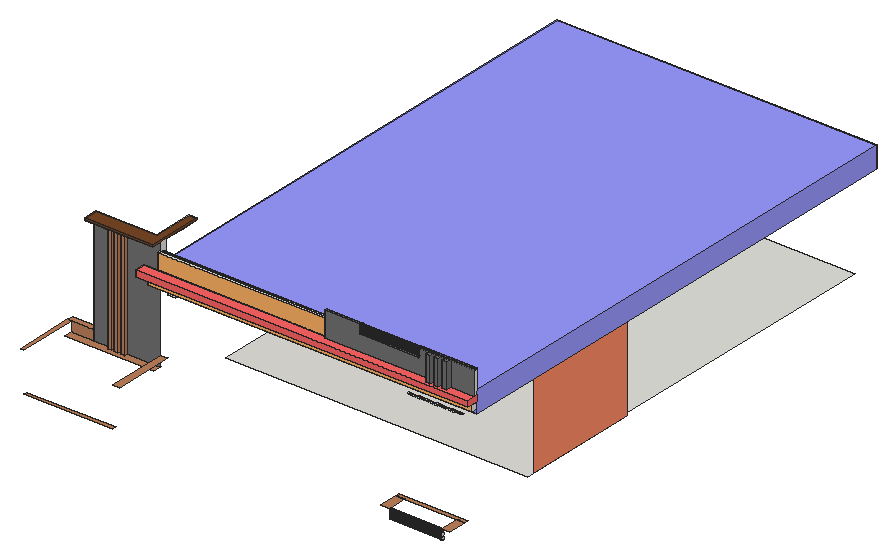
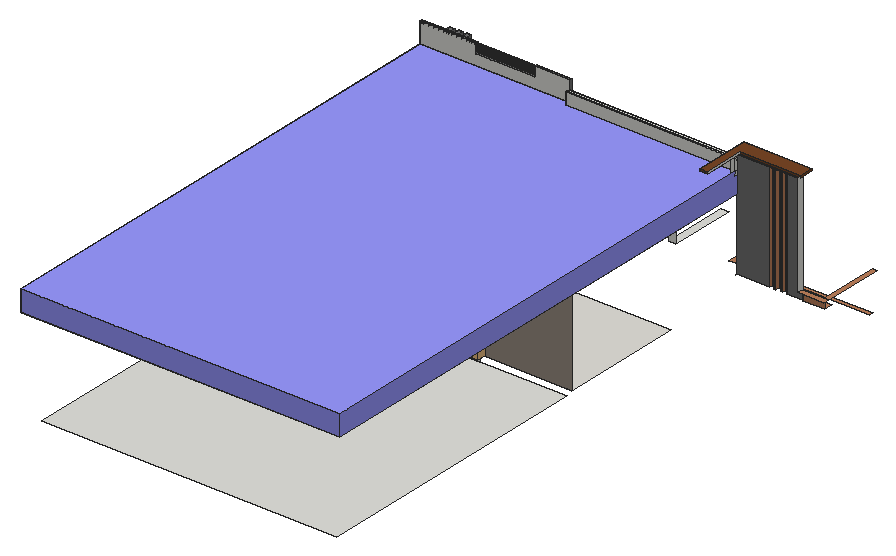
# SketchUp Ruby script. Lengths in inches.
U = 1.inch
M = Sketchup.active_model
def pt(a) = Geom::Point3d.new(a.map { |v| v * U })
def face(e, loops, mat)
  f = e.add_face(loops[0].map { |a| pt(a) })
  loops[1..].each { |l| e.add_face(l.map { |a| pt(a) }).erase! }
  f.material = f.back_material = mat if mat
  f
end
# faces: each face lists its corners as indices into pts; further lists are holes
def faces(e, pts, list, mat = nil) = list.each { |f| face(e, (f[0].is_a?(Array) ? f : [f]).map { |l| l.map { |i| pts[i] } }, mat) }
# xy, xz, yz: faces in a plane at the given z, y or x. An outline is a flat list of corners, or four numbers for a rectangle; further outlines are holes
def ring(l) = l.size == 4 ? [[l[0], l[1]], [l[2], l[1]], [l[2], l[3]], [l[0], l[3]]] : l.each_slice(2).to_a
def flat(e, list, mat, &to3) = list.each { |f| face(e, (f[0].is_a?(Array) ? f : [f]).map { |l| ring(l).map { |u, v| to3.(u, v) } }, mat) }
def xy(e, z, list, mat = nil) = flat(e, list, mat) { |x, y| [x, y, z] }
def xz(e, y, list, mat = nil) = flat(e, list, mat) { |x, z| [x, y, z] }
def yz(e, x, list, mat = nil) = flat(e, list, mat) { |y, z| [x, y, z] }
def lines(e, pts, list) = list.each { |a, b| e.add_line(pt(pts[a]), pt(pts[b])) }
# prism: a flat outline (further loops are holes) pulled along v
def prism(e, loops, v, mat = nil)
  f = face(e, loops, mat); d = Geom::Vector3d.new(v.map { |x| x * U })
  f.pushpull(f.normal.samedirection?(d) ? d.length : -d.length)
end
def box(e, o, s, mat = nil) = prism(e, [[o, [o[0] + s[0], o[1], o[2]], [o[0] + s[0], o[1] + s[1], o[2]], [o[0], o[1] + s[1], o[2]]]], [0, 0, s[2]], mat)
def at(x, y, z, deg = 0) = Geom::Transformation.translation(pt([x, y, z])) * Geom::Transformation.rotation(ORIGIN, Z_AXIS, deg.degrees)
def axes(o, x, y, z) = Geom::Transformation.new([*x, 0, *y, 0, *z, 0, *pt(o).to_a, 1])
def part(name) = M.definitions.add(name)
# library, detail: a bought-in or finely detailed component or shape, given as its bounding box
def library(name, o, s) = part(name).tap { |d| box(d.entities, o, s) }
def detail(e, o, s) = box(e.add_group.entities, o, s)
def put(e, d, t, mat = nil) = e.add_instance(d, t).tap { |i| i.material = mat if mat }
def group(e, t, mat = nil) = e.add_group.tap { |g| g.transformation = t; g.material = mat if mat }.entities
root = M.entities
M.materials.add("[Color A03]").color = [255, 101, 101]
M.materials.add("[Color B03]").color = [255, 140, 101]
M.materials.add("[Color C03]").color = [255, 178, 101]
M.materials.add("[Color I02]").color = [153, 153, 255]
M.materials.add("[Color M05]").color = [114, 114, 114]
M.materials.add("[Marble Carrara Gold Floor Tile]").color = [225, 223, 217]
M.materials.add("[Translucent Glass Gray]1").color = [128, 128, 128]
M.materials["[Translucent Glass Gray]1"].alpha = 0.5
M.materials.add("[Water Stream Shallow]").color = [155, 145, 133]
M.materials.add("[Wood Cherry Original]").color = [152, 86, 42]
M.materials.add("[Wood Veneer 01]").color = [120, 70, 37]
M.materials.add("[Wood Veneer 02]").color = [190, 128, 91]
c1 = library("DOOR (1)",[0,-8.625,0],[36,11.25,84])
c2 = part("Group\#4")
xy(c2.entities,0,[[0,0,32.48,1.97]])
xy(c2.entities,0.98,[[0.98,0,31.5,0.98],[0.98,0.98,31.5,1.97]])
xy(c2.entities,8.86,[[0.98,0,31.5,0.98],[0.98,0.98,31.5,1.97]])
xy(c2.entities,9.84,[[0,0,32.48,1.97]])
xz(c2.entities,0,[[[0,0,32.48,9.84],[0.98,0.98,31.5,8.86]]])
xz(c2.entities,0.98,[[0.98,0.98,31.5,8.86]],"[Translucent Glass Gray]1")
xz(c2.entities,1.97,[[[0,0,32.48,9.84],[0.98,0.98,31.5,8.86]]])
yz(c2.entities,0,[[0,0,1.97,9.84]])
yz(c2.entities,0.98,[[0,0.98,0.98,8.86],[0.98,0.98,1.97,8.86]])
yz(c2.entities,31.5,[[0,0.98,0.98,8.86],[0.98,0.98,1.97,8.86]])
yz(c2.entities,32.48,[[0,0,1.97,9.84]])
c3 = part("Group\#6")
xy(c3.entities,0,[[0,0,32.48,1.97]])
xy(c3.entities,0.98,[[0.98,0,31.5,0.98],[0.98,0.98,31.5,1.97]])
xy(c3.entities,71.85,[[0.98,0,31.5,0.98],[0.98,0.98,31.5,1.97]])
xy(c3.entities,72.83,[[0,0,32.48,1.97]])
xz(c3.entities,0,[[[0,0,32.48,72.83],[0.98,0.98,31.5,71.85]]])
xz(c3.entities,0.98,[[0.98,0.98,31.5,71.85]],"[Translucent Glass Gray]1")
xz(c3.entities,1.97,[[[0,0,32.48,72.83],[0.98,0.98,31.5,71.85]]])
yz(c3.entities,0,[[0,0,1.97,72.83]])
yz(c3.entities,0.98,[[0,0.98,0.98,71.85],[0.98,0.98,1.97,71.85]])
yz(c3.entities,31.5,[[0,0.98,0.98,71.85],[0.98,0.98,1.97,71.85]])
yz(c3.entities,32.48,[[0,0,1.97,72.83]])
c4 = part("FIXED+GLASS+WINDOW+WITH+TRANSOM")
g1 = group(c4.entities,at(0,7.5625,-3.14))
xy(g1,0,[[0,-3.73,93.63,0]])
xy(g1,2.39,[[2.6,-3.73,45.52,-2.8],[48.12,-3.73,91.03,0],[2.6,-0.93,45.52,0]])
xy(g1,105.27,[[2.6,-3.73,45.52,0],[45.52,-3.73,48.12,0],[48.12,-3.73,91.03,0]])
xy(g1,107.66,[[0,-3.73,93.63,0]])
xz(g1,-3.73,[[[0,0,93.63,107.66],[2.6,2.39,45.52,105.27],[48.12,2.39,91.03,105.27]]])
xz(g1,0,[[[0,0,93.63,107.66],[2.6,2.39,45.52,105.27],[48.12,2.39,91.03,105.27]]])
yz(g1,0,[[-3.73,0,0,107.66]])
yz(g1,2.6,[[-3.73,2.39,0,90.92],[-3.73,93.31,0,105.27]])
yz(g1,45.52,[[-3.73,2.39,0,105.27]])
yz(g1,48.12,[[-3.73,2.39,0,105.27]])
yz(g1,91.03,[[-3.73,2.39,0,105.27]])
yz(g1,93.63,[[-3.73,0,0,107.66]])
g2 = group(g1,at(2.6,0,90.92))
box(g2,[0,-3.73,0],[88.43,3.73,2.39])
put(g1,c2,axes([2.6,-0.93,93.31],[1.32132,0,0],[0,-0.94801,0],[0,0,1.2154]))
put(g1,c2,axes([48.12,-0.93,93.31],[1.32132,0,0],[0,-0.94801,0],[0,0,1.2154]))
put(g1,c3,axes([2.6,-0.93,2.39],[1.32132,0,0],[0,-0.94801,0],[0,0,1.2154]))
put(g1,c3,axes([48.12,-0.93,2.39],[1.32132,0,0],[0,-0.94801,0],[0,0,1.2154]))
xy(root,5.125,[[4.34,0,104.79,4.19]],"[Wood Veneer 02]")
xy(root,11.625,[[114.76,294.58,448.89,619.58]])
xy(root,14.625,[[386.33,27.35,395.89,48.85]],"[Wood Veneer 02]")
xy(root,14.6875,[[386.33,48.85,464.58,53.1]],"[Wood Veneer 02]")
xy(root,14.91,[[455.01,27.35,464.58,48.85]],"[Wood Veneer 02]")
xy(root,15,[[113.7,148.58,455.7,148.58,455.7,288.58,248.89,288.58,248.89,294.58,212.89,294.58,212.89,288.58,113.7,288.58]],"[Marble Carrara Gold Floor Tile]")
xy(root,38.8125,[[4.34,57.44,104.79,57.44,104.79,67.36,104.7,67.36,104.7,66.64,67.79,66.64,67.79,63.64,63.1,63.64,63.1,66.64,59.98,66.64,59.98,63.64,55.29,63.64,55.29,66.64,52.61,66.64,52.61,63.64,47.91,63.64,47.91,66.64,29.5,66.64,29.5,67.36,4.34,67.36]],"[Wood Veneer 02]")
xy(root,41.07,[[327.66,288.58,375.66,294.58]])
xy(root,50,[[0,0,4.34,67.36],[104.79,0,112.66,67.32],[0,67.36,29.5,73.72]],"[Wood Veneer 02]")
xy(root,84,[[212.89,288.58,248.89,294.58]])
xy(root,89.07,[[327.66,288.58,375.66,294.58]])
xy(root,107.35,[[104.79,78.01,113.42,152.44]])
xy(root,120,[[[455.7,65.3,464.7,65.3,464.7,628.58,104.7,628.58,104.7,148.58,110.64,148.58,110.64,78.01,113.7,78.01,113.7,288.58,455.7,288.58],[113.7,294.58,455.7,619.58]],[104.7,66.64,106.01,73.72],[104.7,73.72,106.01,148.58],[106.01,73.72,110.64,148.58]])
xy(root,121.125,[[104.79,67.32,113.42,152.44]])
xy(root,124.36,[[99.19,57.01,466.06,63.01]])
xy(root,130.99,[[99.19,57.01,466.06,63.01]])
xy(root,132,[[89.58,51.01,466.14,63.01]],"[Wood Cherry Original]")
xy(root,138.625,[[415.41,54.01,420.69,60.01],[424.66,54.01,429.94,60.01],[433.91,54.01,439.19,60.01],[297.02,60.01,342.89,63.01],[342.89,60.01,466.08,63.01],
  [104.95,63.01,297.02,66.01],[104.95,66.01,297.02,68.39]])
xy(root,138.625,[[89.58,51.01,466.14,51.01,466.14,63.01,466.08,63.01,466.08,60.01,439.19,60.01,439.19,54.01,433.91,54.01,433.91,60.01,429.94,60.01,429.94,54.01,424.66,54.01,424.66,60.01,420.69,60.01,420.69,54.01,415.41,54.01,415.41,60.01,297.02,60.01,297.02,63.01,89.58,63.01]],"[Color A03]")
xy(root,156,[[335.91,60.01,403.1,63.01]],"[Color M05]")
xy(root,156.51,[[104.95,63.01,297.02,66.01],[104.95,66.01,297.02,68.39]])
xy(root,165.75,[[28.39,55.2,29.5,71.95],[29.5,55.2,47.91,66.64],[47.91,55.2,52.61,63.64],[52.61,55.2,55.29,66.64],[55.29,55.2,59.98,63.64],
  [59.98,55.2,63.1,66.64],[63.1,55.2,67.79,63.64],[67.79,55.2,106.01,66.64],[47.91,63.64,52.61,66.64],[55.29,63.64,59.98,66.64],
  [63.1,63.64,67.79,66.64],[29.5,66.64,106.01,71.95],[29.5,71.95,96.84,73.72],[96.84,71.95,106.01,73.72],[96.84,73.72,106.01,76.7],
  [96.84,76.7,106.01,102.95],[96.84,102.95,106.01,117.33]])
xy(root,166.75,[[415.41,54.01,420.69,60.01],[424.66,54.01,429.94,60.01],[433.91,54.01,439.19,60.01],[297.02,60.01,335.91,63.01],[403.1,60.01,466.08,63.01]],"[Color M05]")
xy(root,167.75,[[28.39,55.2,106.01,55.2,106.01,117.33,96.84,117.33,96.84,71.95,28.39,71.95]],"[Wood Veneer 01]")
xz(root,48.85,[[386.33,14.625,395.89,14.6875],[455.01,14.6875,464.58,14.91]])
xz(root,51.01,[[89.58,132,466.14,138.625]],"[Color A03]")
xz(root,54.01,[[415.41,138.625,420.69,166.75],[424.66,138.625,429.94,166.75],[433.91,138.625,439.19,166.75]],"[Color M05]")
xz(root,55.2,[[28.39,165.75,106.01,167.75]],"[Wood Veneer 01]")
xz(root,57.01,[[99.19,124.36,466.06,130.99]],"[Color C03]")
xz(root,60.01,[[415.41,138.625,420.69,166.75],[424.66,138.625,429.94,166.75],[433.91,138.625,439.19,166.75]])
xz(root,60.01,[[297.02,138.625,415.41,138.625,415.41,166.75,403.1,166.75,403.1,156,335.91,156,335.91,166.75,297.02,166.75],[420.69,138.625,424.66,166.75],[429.94,138.625,433.91,166.75],[439.19,138.625,466.08,166.75]],"[Color M05]")
xz(root,63.01,[[99.19,124.36,466.06,130.99],[89.58,132,104.95,138.625],[104.95,132,342.89,138.625],[342.89,132,466.14,138.625],[297.02,138.625,297.02,166.75,335.91,166.75,335.91,156,403.1,156,403.1,166.75,466.08,166.75,466.08,138.625]])
xz(root,63.01,[[104.95,138.625,297.02,156.51]],"[Color C03]")
xz(root,63.64,[[47.91,38.8125,52.61,165.75],[55.29,38.8125,59.98,165.75],[63.1,38.8125,67.79,165.75]],"[Wood Veneer 02]")
xz(root,66.64,[[29.5,38.8125,47.91,165.75],[52.61,38.8125,55.29,165.75],[59.98,38.8125,63.1,165.75],[67.79,38.8125,104.7,38.8125,104.7,120,106.01,120,106.01,165.75,67.79,165.75]],"[Color M05]")
xz(root,67.36,[[4.34,38.8125,29.5,50]],"[Wood Veneer 02]")
xz(root,68.39,[[104.95,138.625,297.02,156.51]])
xz(root,71.95,[[28.39,165.75,96.84,167.75]],"[Wood Veneer 01]")
xz(root,117.33,[[96.84,165.75,106.01,167.75]],"[Wood Veneer 01]")
xz(root,152.44,[[104.79,107.35,113.42,121.125]])
xz(root,288.58,[[[113.7,15,212.89,15,212.89,84,248.89,84,248.89,15,455.7,15,455.7,120,113.7,120],[327.66,41.07,375.66,89.07]]],"[Water Stream Shallow]")
xz(root,294.58,[[212.89,11.625,248.89,15]])
yz(root,28.39,[[55.2,165.75,71.95,167.75]],"[Wood Veneer 01]")
yz(root,29.5,[[66.64,38.8125,66.64,165.75,73.72,165.75,73.72,50,67.36,50,67.36,38.8125]])
yz(root,47.91,[[63.64,38.8125,66.64,165.75]],"[Wood Veneer 02]")
yz(root,52.61,[[63.64,38.8125,66.64,165.75]],"[Wood Veneer 02]")
yz(root,55.29,[[63.64,38.8125,66.64,165.75]],"[Wood Veneer 02]")
yz(root,59.98,[[63.64,38.8125,66.64,165.75]],"[Wood Veneer 02]")
yz(root,63.1,[[63.64,38.8125,66.64,165.75]],"[Wood Veneer 02]")
yz(root,67.79,[[63.64,38.8125,66.64,165.75]],"[Wood Veneer 02]")
yz(root,89.58,[[51.01,132,63.01,138.625]],"[Color A03]")
yz(root,96.84,[[71.95,165.75,117.33,167.75]])
yz(root,99.19,[[57.01,124.36,63.01,130.99]])
yz(root,104.95,[[63.01,138.625,68.39,144],[63.01,144,66.01,156.51],[66.01,144,68.39,156.51]])
yz(root,106.01,[[66.64,120,73.72,165.75]])
yz(root,106.01,[[55.2,165.75,117.33,167.75]],"[Wood Veneer 01]")
yz(root,212.89,[[288.58,15,294.58,84]])
yz(root,248.89,[[288.58,15,294.58,84]])
yz(root,297.02,[[63.01,138.625,66.01,144],[66.01,138.625,68.39,144],[63.01,144,66.01,156.51],[66.01,144,68.39,156.51]])
yz(root,297.02,[[60.01,138.625,63.01,166.75]],"[Color M05]")
yz(root,327.66,[[288.58,41.07,294.58,89.07]])
yz(root,335.91,[[[60.01,156,63.01,166.75],[61.38,164.68,61.125,164.71,60.88,164.8125,60.68,164.97,60.52,165.18,60.42,165.42,60.38,165.68,60.42,165.9375,60.52,166.18,60.68,166.39,60.88,166.55,61.125,166.65,61.38,166.68,61.64,166.65,61.88,166.55,62.09,166.39,62.25,166.18,62.35,165.9375,62.38,165.68,62.35,165.42,62.25,165.18,62.09,164.97,61.88,164.8125,61.64,164.71],[61.38,161.43,61.125,161.46,60.88,161.5625,60.68,161.72,60.52,161.93,60.42,162.17,60.38,162.43,60.42,162.6875,60.52,162.93,60.68,163.14,60.88,163.3,61.125,163.4,61.38,163.43,61.64,163.4,61.88,163.3,62.09,163.14,62.25,162.93,62.35,162.6875,62.38,162.43,62.35,162.17,62.25,161.93,62.09,161.72,61.88,161.5625,61.64,161.46],[61.38,157.68,61.125,157.71,60.88,157.8125,60.68,157.97,60.52,158.18,60.42,158.42,60.38,158.68,60.42,158.9375,60.52,159.18,60.68,159.39,60.88,159.55,61.125,159.65,61.38,159.68,61.64,159.65,61.88,159.55,62.09,159.39,62.25,159.18,62.35,158.9375,62.38,158.68,62.35,158.42,62.25,158.18,62.09,157.97,61.88,157.8125,61.64,157.71]]],"[Color M05]")
yz(root,375.66,[[288.58,41.07,294.58,89.07]])
yz(root,395.89,[[28.97,3.38,28.61,3.43,28.28,3.57,28,3.78,27.78,4.07,27.64,4.4,27.59,4.76,27.64,5.11,27.78,5.44,28,5.73,28.28,5.95,28.61,6.09,28.97,6.13,29.32,6.09,29.66,5.95,29.94,5.73,30.16,5.44,30.3,5.11,30.34,4.76,30.3,4.4,30.16,4.07,29.94,3.78,29.66,3.57,29.32,3.43],[28.97,7.19,28.61,7.24,28.28,7.38,28,7.6,27.78,7.88,27.64,8.21,27.59,8.57,27.64,8.93,27.78,9.26,28,9.54,28.28,9.76,28.61,9.9,28.97,9.94,29.32,9.9,29.66,9.76,29.94,9.54,30.16,9.26,30.3,8.93,30.34,8.57,30.3,8.21,30.16,7.88,29.94,7.6,29.66,7.38,29.32,7.24],[28.97,11.57,28.61,11.62,28.28,11.75,28,11.97,27.78,12.26,27.64,12.59,27.59,12.94,27.64,13.3,27.78,13.63,28,13.92,28.28,14.14,28.61,14.27,28.97,14.32,29.32,14.27,29.66,14.14,29.94,13.92,30.16,13.63,30.3,13.3,30.34,12.94,30.3,12.59,30.16,12.26,29.94,11.97,29.66,11.75,29.32,11.62]])
yz(root,403.1,[[[60.01,156,63.01,166.75],[61.38,161.43,61.64,161.46,61.88,161.5625,62.09,161.72,62.25,161.93,62.35,162.17,62.38,162.43,62.35,162.6875,62.25,162.93,62.09,163.14,61.88,163.3,61.64,163.4,61.38,163.43,61.125,163.4,60.88,163.3,60.68,163.14,60.52,162.93,60.42,162.6875,60.38,162.43,60.42,162.17,60.52,161.93,60.68,161.72,60.88,161.5625,61.125,161.46]]],"[Color M05]")
yz(root,404.16,[[61.38,157.68,61.64,157.71,61.88,157.8125,62.09,157.97,62.25,158.18,62.35,158.42,62.38,158.68,62.35,158.9375,62.25,159.18,62.09,159.39,61.88,159.55,61.64,159.65,61.38,159.68,61.125,159.65,60.88,159.55,60.68,159.39,60.52,159.18,60.42,158.9375,60.38,158.68,60.42,158.42,60.52,158.18,60.68,157.97,60.88,157.8125,61.125,157.71]])
yz(root,415.41,[[54.01,138.625,60.01,166.75]],"[Color M05]")
yz(root,420.69,[[54.01,138.625,60.01,166.75]],"[Color M05]")
yz(root,424.66,[[54.01,138.625,60.01,166.75]],"[Color M05]")
yz(root,429.94,[[54.01,138.625,60.01,166.75]],"[Color M05]")
yz(root,433.91,[[54.01,138.625,60.01,166.75]],"[Color M05]")
yz(root,439.19,[[54.01,138.625,60.01,166.75]],"[Color M05]")
yz(root,455.26,[[28.97,7.19,29.32,7.24,29.66,7.38,29.94,7.6,30.16,7.88,30.3,8.21,30.34,8.57,30.3,8.93,30.16,9.26,29.94,9.54,29.66,9.76,29.32,9.9,28.97,9.94,28.61,9.9,28.28,9.76,28,9.54,27.78,9.26,27.64,8.93,27.59,8.57,27.64,8.21,27.78,7.88,28,7.6,28.28,7.38,28.61,7.24]])
yz(root,455.51,[[28.97,3.38,29.32,3.43,29.66,3.57,29.94,3.78,30.16,4.07,30.3,4.4,30.34,4.76,30.3,5.11,30.16,5.44,29.94,5.73,29.66,5.95,29.32,6.09,28.97,6.13,28.61,6.09,28.28,5.95,28,5.73,27.78,5.44,27.64,5.11,27.59,4.76,27.64,4.4,27.78,4.07,28,3.78,28.28,3.57,28.61,3.43]])
yz(root,455.7,[[157.58,15,288.58,120]],"[Color B03]")
yz(root,466.06,[[57.01,124.36,63.01,130.99]])
yz(root,466.08,[[60.01,138.625,63.01,166.75]])
yz(root,466.14,[[61.38,164.68,61.64,164.71,61.88,164.8125,62.09,164.97,62.25,165.18,62.35,165.42,62.38,165.68,62.35,165.9375,62.25,166.18,62.09,166.39,61.88,166.55,61.64,166.65,61.38,166.68,61.125,166.65,60.88,166.55,60.68,166.39,60.52,166.18,60.42,165.9375,60.38,165.68,60.42,165.42,60.52,165.18,60.68,164.97,60.88,164.8125,61.125,164.71]])
yz(root,466.14,[[51.01,132,63.01,138.625]],"[Color A03]")
p = [[395.89,28.28,3.57],[395.89,28.61,3.43],[455.51,28.61,3.43],[455.51,28.28,3.57],[395.89,28.97,3.38],[455.51,28.97,3.38],
  [395.89,29.32,3.43],[455.51,29.32,3.43],[395.89,29.66,3.57],[455.51,29.66,3.57],[395.89,28,3.78],[455.51,28,3.78],
  [395.89,29.94,3.78],[455.51,29.94,3.78],[395.89,27.78,4.07],[455.51,27.78,4.07],[395.89,30.16,4.07],[455.51,30.16,4.07],
  [395.89,27.64,4.4],[455.51,27.64,4.4],[395.89,30.3,4.4],[455.51,30.3,4.4],[395.89,27.59,4.76],[455.51,27.59,4.76],
  [395.89,30.34,4.76],[455.51,30.34,4.76],[395.89,27.64,5.11],[455.51,27.64,5.11],[395.89,30.3,5.11],[455.51,30.3,5.11],
  [395.89,27.78,5.44],[455.51,27.78,5.44],[395.89,30.16,5.44],[455.51,30.16,5.44],[395.89,28,5.73],[455.51,28,5.73],
  [395.89,29.94,5.73],[455.51,29.94,5.73],[395.89,28.28,5.95],[455.51,28.28,5.95],[395.89,29.66,5.95],[455.51,29.66,5.95],
  [395.89,28.61,6.09],[455.51,28.61,6.09],[395.89,29.32,6.09],[455.51,29.32,6.09],[395.89,28.97,6.13],[455.51,28.97,6.13],
  [395.89,28.28,7.38],[395.89,28.61,7.24],[455.26,28.61,7.24],[455.26,28.28,7.38],[395.89,28.97,7.19],[455.26,28.97,7.19],
  [395.89,29.32,7.24],[455.26,29.32,7.24],[395.89,29.66,7.38],[455.26,29.66,7.38],[395.89,28,7.6],[455.26,28,7.6],
  [395.89,29.94,7.6],[455.26,29.94,7.6],[395.89,27.78,7.88],[455.26,27.78,7.88],[395.89,30.16,7.88],[455.26,30.16,7.88],
  [395.89,27.64,8.21],[455.26,27.64,8.21],[395.89,30.3,8.21],[455.26,30.3,8.21],[395.89,27.59,8.57],[455.26,27.59,8.57],
  [395.89,30.34,8.57],[455.26,30.34,8.57],[395.89,27.64,8.93],[455.26,27.64,8.93],[395.89,30.3,8.93],[455.26,30.3,8.93],
  [395.89,27.78,9.26],[455.26,27.78,9.26],[395.89,30.16,9.26],[455.26,30.16,9.26],[395.89,28,9.54],[455.26,28,9.54],
  [395.89,29.94,9.54],[455.26,29.94,9.54],[395.89,28.28,9.76],[455.26,28.28,9.76],[395.89,29.66,9.76],[455.26,29.66,9.76],
  [395.89,28.61,9.9],[455.26,28.61,9.9],[395.89,29.32,9.9],[455.26,29.32,9.9],[395.89,28.97,9.94],[455.26,28.97,9.94],
  [395.89,28.28,11.75],[395.89,28.61,11.62],[455.01,28.61,11.62],[455.01,28.28,11.75],[395.89,28.97,11.57],[455.01,28.97,11.57],
  [395.89,29.32,11.62],[455.01,29.32,11.62],[395.89,29.66,11.75],[455.01,29.66,11.75],[395.89,28,11.97],[455.01,28,11.97],
  [395.89,29.94,11.97],[455.01,29.94,11.97],[395.89,27.78,12.26],[455.01,27.78,12.26],[395.89,30.16,12.26],[455.01,30.16,12.26],
  [395.89,27.64,12.59],[455.01,27.64,12.59],[395.89,30.3,12.59],[455.01,30.3,12.59],[395.89,27.59,12.94],[455.01,27.59,12.94],
  [395.89,30.34,12.94],[455.01,30.34,12.94],[395.89,27.64,13.3],[455.01,27.64,13.3],[395.89,30.3,13.3],[455.01,30.3,13.3],
  [395.89,27.78,13.63],[455.01,27.78,13.63],[395.89,30.16,13.63],[455.01,30.16,13.63],[395.89,28,13.92],[455.01,28,13.92],
  [395.89,29.94,13.92],[455.01,29.94,13.92],[395.89,28.28,14.14],[455.01,28.28,14.14],[395.89,29.66,14.14],[455.01,29.66,14.14],
  [395.89,28.61,14.27],[455.01,28.61,14.27],[395.89,29.32,14.27],[455.01,29.32,14.27],[395.89,28.97,14.32],[455.01,28.97,14.32],
  [395.375,56.92,118.16],[392.875,56.92,118.16],[392.875,58.48,118.13],[395.375,58.48,118.13],[397.875,56.92,118.16],[397.875,58.48,118.13],
  [400.375,56.92,118.16],[400.375,58.48,118.13],[402.875,56.92,118.16],[402.875,58.48,118.13],[405.375,56.92,118.16],[405.375,58.48,118.13],
  [407.875,56.92,118.16],[407.875,58.48,118.13],[410.375,56.92,118.16],[410.375,58.48,118.13],[412.875,56.92,118.16],[412.875,58.48,118.13],
  [415.375,56.92,118.16],[415.375,58.48,118.13],[417.875,56.92,118.16],[417.875,58.48,118.13],[420.375,56.92,118.16],[420.375,58.48,118.13],
  [422.875,56.92,118.16],[422.875,58.48,118.13],[425.375,56.92,118.16],[425.375,58.48,118.13],[427.875,56.92,118.16],[427.875,58.48,118.13],
  [430.375,56.92,118.16],[430.375,58.48,118.13],[432.875,56.92,118.16],[432.875,58.48,118.13],[435.375,56.92,118.16],[435.375,58.48,118.13],
  [437.875,56.92,118.16],[437.875,58.48,118.13],[440.375,56.92,118.16],[440.375,58.48,118.13],[442.875,56.92,118.16],[442.875,58.48,118.13],
  [445.375,56.92,118.16],[445.375,58.48,118.13],[447.875,56.92,118.16],[447.875,58.48,118.13],[450.375,56.92,118.16],[450.375,58.48,118.13],
  [450.45,58.48,118.13],[452.875,58.48,118.13],[452.875,56.92,118.16],[450.45,56.92,118.16],[454.76,56.92,118.16],[454.76,58.48,118.13],
  [397.875,55.48,118.18],[395.375,55.48,118.18],[402.875,55.48,118.18],[400.375,55.48,118.18],[407.875,55.48,118.18],[405.375,55.48,118.18],
  [412.875,55.48,118.18],[410.375,55.48,118.18],[417.875,55.48,118.18],[415.375,55.48,118.18],[422.875,55.48,118.18],[420.375,55.48,118.18],
  [427.875,55.48,118.18],[425.375,55.48,118.18],[432.875,55.48,118.18],[430.375,55.48,118.18],[437.875,55.48,118.18],[435.375,55.48,118.18],
  [442.875,55.48,118.18],[440.375,55.48,118.18],[447.875,55.48,118.18],[445.375,55.48,118.18],[450.45,55.48,118.18],[450.375,55.48,118.18],
  [452.875,55.48,118.18],[454.76,63.01,124.36],[462.78,63.01,124.36],[462.78,151.07,122.96],[454.76,151.07,122.96],[450.45,63.01,124.36],
  [401.32,63.01,124.36],[390.38,63.01,124.36],[390.38,57.02,124.46],[450.45,57.02,124.46],[390.38,57.01,124.36],[450.45,57.01,124.36],
  [454.76,57.02,124.46],[454.76,57.01,124.36],[462.78,57.02,124.46],[462.78,57.01,124.36],[335.91,60.88,157.8125],[335.91,61.125,157.71],
  [404.16,61.125,157.71],[404.16,60.88,157.8125],[335.91,61.38,157.68],[404.16,61.38,157.68],[335.91,61.64,157.71],[404.16,61.64,157.71],
  [335.91,61.88,157.8125],[404.16,61.88,157.8125],[335.91,60.68,157.97],[404.16,60.68,157.97],[335.91,62.09,157.97],[404.16,62.09,157.97],
  [335.91,60.52,158.18],[404.16,60.52,158.18],[335.91,62.25,158.18],[404.16,62.25,158.18],[335.91,60.42,158.42],[404.16,60.42,158.42],
  [335.91,62.35,158.42],[404.16,62.35,158.42],[335.91,60.38,158.68],[404.16,60.38,158.68],[335.91,62.38,158.68],[404.16,62.38,158.68],
  [335.91,60.42,158.9375],[404.16,60.42,158.9375],[335.91,62.35,158.9375],[404.16,62.35,158.9375],[335.91,60.52,159.18],[404.16,60.52,159.18],
  [335.91,62.25,159.18],[404.16,62.25,159.18],[335.91,60.68,159.39],[404.16,60.68,159.39],[335.91,62.09,159.39],[404.16,62.09,159.39],
  [335.91,60.88,159.55],[404.16,60.88,159.55],[335.91,61.88,159.55],[404.16,61.88,159.55],[335.91,61.125,159.65],[404.16,61.125,159.65],
  [335.91,61.64,159.65],[404.16,61.64,159.65],[335.91,61.38,159.68],[404.16,61.38,159.68],[335.91,61.125,161.46],[335.91,61.38,161.43],
  [403.1,61.38,161.43],[403.1,61.125,161.46],[335.91,61.64,161.46],[403.1,61.64,161.46],[335.91,60.88,161.5625],[403.1,60.88,161.5625],
  [335.91,61.88,161.5625],[403.1,61.88,161.5625],[335.91,60.68,161.72],[403.1,60.68,161.72],[335.91,62.09,161.72],[403.1,62.09,161.72],
  [335.91,60.52,161.93],[403.1,60.52,161.93],[335.91,62.25,161.93],[403.1,62.25,161.93],[335.91,60.42,162.17],[403.1,60.42,162.17],
  [335.91,62.35,162.17],[403.1,62.35,162.17],[335.91,60.38,162.43],[403.1,60.38,162.43],[335.91,62.38,162.43],[403.1,62.38,162.43],
  [335.91,60.42,162.6875],[403.1,60.42,162.6875],[335.91,62.35,162.6875],[403.1,62.35,162.6875],[335.91,60.52,162.93],[403.1,60.52,162.93],
  [335.91,62.25,162.93],[403.1,62.25,162.93],[335.91,60.68,163.14],[403.1,60.68,163.14],[335.91,62.09,163.14],[403.1,62.09,163.14],
  [335.91,60.88,163.3],[403.1,60.88,163.3],[335.91,61.88,163.3],[403.1,61.88,163.3],[335.91,61.125,163.4],[403.1,61.125,163.4],
  [335.91,61.64,163.4],[403.1,61.64,163.4],[335.91,61.38,163.43],[403.1,61.38,163.43],[335.91,60.88,164.8125],[335.91,61.125,164.71],
  [466.14,61.125,164.71],[466.14,60.88,164.8125],[335.91,61.38,164.68],[466.14,61.38,164.68],[335.91,61.64,164.71],[466.14,61.64,164.71],
  [335.91,61.88,164.8125],[466.14,61.88,164.8125],[335.91,60.68,164.97],[466.14,60.68,164.97],[335.91,62.09,164.97],[466.14,62.09,164.97],
  [335.91,60.52,165.18],[466.14,60.52,165.18],[335.91,62.25,165.18],[466.14,62.25,165.18],[335.91,60.42,165.42],[466.14,60.42,165.42],
  [335.91,62.35,165.42],[466.14,62.35,165.42],[335.91,60.38,165.68],[466.14,60.38,165.68],[335.91,62.38,165.68],[466.14,62.38,165.68],
  [335.91,60.42,165.9375],[466.14,60.42,165.9375],[335.91,62.35,165.9375],[466.14,62.35,165.9375],[335.91,60.52,166.18],[466.14,60.52,166.18],
  [335.91,62.25,166.18],[466.14,62.25,166.18],[335.91,60.68,166.39],[466.14,60.68,166.39],[335.91,62.09,166.39],[466.14,62.09,166.39],
  [335.91,60.88,166.55],[466.14,60.88,166.55],[335.91,61.88,166.55],[466.14,61.88,166.55],[335.91,61.125,166.65],[466.14,61.125,166.65],
  [335.91,61.64,166.65],[466.14,61.64,166.65],[335.91,61.38,166.68],[466.14,61.38,166.68],[466.14,63.01,120]]
faces(root,p,[[0,1,2,3],[1,4,5,2],[4,6,7,5],[6,8,9,7],[10,0,3,11],[8,12,13,9],[14,10,11,15],[12,16,17,13],
  [18,14,15,19],[16,20,21,17],[22,18,19,23],[20,24,25,21],[26,22,23,27],[24,28,29,25],[30,26,27,31],[28,32,33,29],
  [34,30,31,35],[32,36,37,33],[38,34,35,39],[36,40,41,37],[42,38,39,43],[40,44,45,41],[46,42,43,47],[44,46,47,45],
  [48,49,50,51],[49,52,53,50],[52,54,55,53],[54,56,57,55],[58,48,51,59],[56,60,61,57],[62,58,59,63],[60,64,65,61],
  [66,62,63,67],[64,68,69,65],[70,66,67,71],[68,72,73,69],[74,70,71,75],[72,76,77,73],[78,74,75,79],[76,80,81,77],
  [82,78,79,83],[80,84,85,81],[86,82,83,87],[84,88,89,85],[90,86,87,91],[88,92,93,89],[94,90,91,95],[92,94,95,93],
  [96,97,98,99],[97,100,101,98],[100,102,103,101],[102,104,105,103],[106,96,99,107],[104,108,109,105],[110,106,107,111],[108,112,113,109],
  [114,110,111,115],[112,116,117,113],[118,114,115,119],[116,120,121,117],[122,118,119,123],[120,124,125,121],[126,122,123,127],[124,128,129,125],
  [130,126,127,131],[128,132,133,129],[134,130,131,135],[132,136,137,133],[138,134,135,139],[136,140,141,137],[142,138,139,143],[140,142,143,141],
  [238,239,240,241],[239,242,243,240],[242,244,245,243],[244,246,247,245],[248,238,241,249],[246,250,251,247],[252,248,249,253],[250,254,255,251],
  [256,252,253,257],[254,258,259,255],[260,256,257,261],[258,262,263,259],[264,260,261,265],[262,266,267,263],[268,264,265,269],[266,270,271,267],
  [272,268,269,273],[270,274,275,271],[276,272,273,277],[274,278,279,275],[280,276,277,281],[278,282,283,279],[284,280,281,285],[282,284,285,283],
  [286,287,288,289],[287,290,291,288],[292,286,289,293],[290,294,295,291],[296,292,293,297],[294,298,299,295],[300,296,297,301],[298,302,303,299],
  [304,300,301,305],[302,306,307,303],[308,304,305,309],[306,310,311,307],[312,308,309,313],[310,314,315,311],[316,312,313,317],[314,318,319,315],
  [320,316,317,321],[318,322,323,319],[324,320,321,325],[322,326,327,323],[328,324,325,329],[326,330,331,327],[332,328,329,333],[330,332,333,331],
  [334,335,336,337],[335,338,339,336],[338,340,341,339],[340,342,343,341],[344,334,337,345],[342,346,347,343],[348,344,345,349],[346,350,351,347],
  [352,348,349,353],[350,354,355,351],[356,352,353,357],[354,358,359,355],[360,356,357,361],[358,362,363,359],[364,360,361,365],[362,366,367,363],
  [368,364,365,369],[366,370,371,367],[372,368,369,373],[370,374,375,371],[376,372,373,377],[374,378,379,375],[380,376,377,381],[378,380,381,379]],"[Color M05]")
faces(root,p,[[144,145,146,147],[148,144,147,149],[150,148,149,151],[152,150,151,153],[154,152,153,155],[156,154,155,157],[158,156,157,159],[160,158,159,161],
  [162,160,161,163],[164,162,163,165],[166,164,165,167],[168,166,167,169],[170,168,169,171],[172,170,171,173],[174,172,173,175],[176,174,175,177],
  [178,176,177,179],[180,178,179,181],[182,180,181,183],[184,182,183,185],[186,184,185,187],[188,186,187,189],[190,188,189,191],[192,193,194,195],
  [195,190,191,192],[196,194,193,197],[198,148,144,199],[200,152,150,201],[202,156,154,203],[204,160,158,205],[206,164,162,207],[208,168,166,209],
  [210,172,170,211],[212,176,174,213],[214,180,178,215],[216,184,182,217],[218,188,186,219],[220,195,190,221],[222,194,195,220],[223,224,225,226],
  [227,228,229,230,231],[232,233,231,230],[231,234,223,227],[233,235,234,231],[224,223,234,236],[236,234,235,237]])
lines(root,p,[[382,196]])
put(root,c1,axes([212.89,295.19,15],[1,0,0],[0,0.76667,0],[0,0,0.82143]))
put(root,c4,axes([327.66,288.58,41.07],[0.52801,0,0],[0,0.45518,0],[0,0,0.45518]))
g3 = group(root,at(113.7,148.58,120),"[Color I02]")
box(g3,[-8.75,-85.5625,0],[361.1875,565.625,24])
